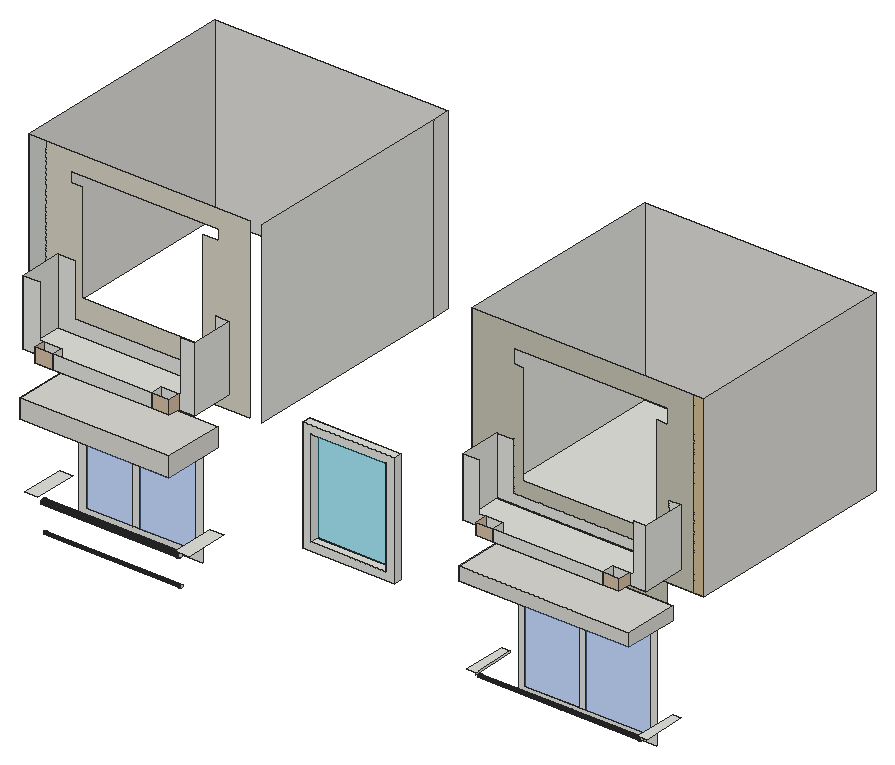
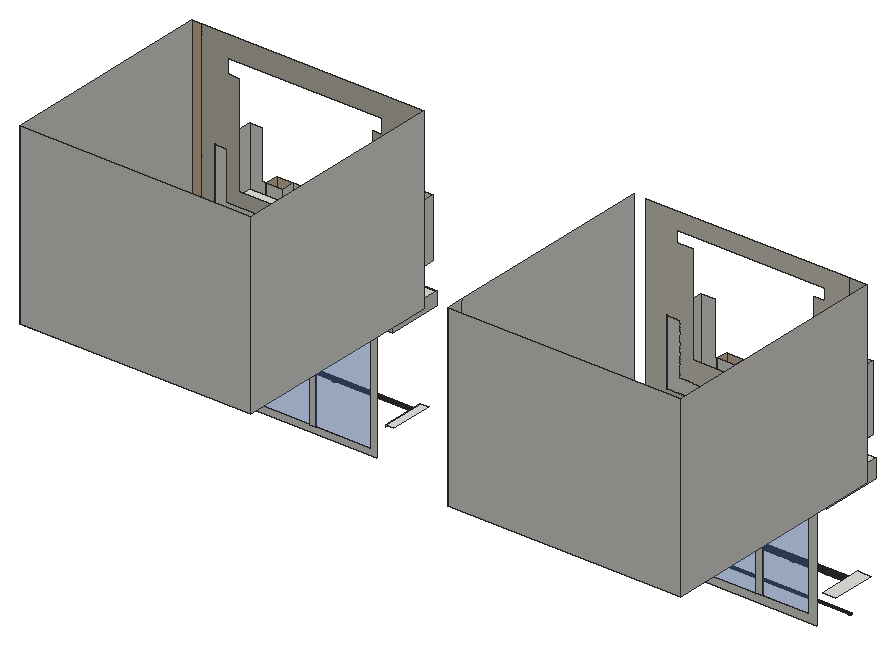
# SketchUp Ruby script. Lengths in inches.
U = 1.inch
M = Sketchup.active_model
def pt(a) = Geom::Point3d.new(a.map { |v| v * U })
def face(e, loops, mat)
  f = e.add_face(loops[0].map { |a| pt(a) })
  loops[1..].each { |l| e.add_face(l.map { |a| pt(a) }).erase! }
  f.material = f.back_material = mat if mat
  f
end
# faces: each face lists its corners as indices into pts; further lists are holes
def faces(e, pts, list, mat = nil) = list.each { |f| face(e, (f[0].is_a?(Array) ? f : [f]).map { |l| l.map { |i| pts[i] } }, mat) }
# xy, xz, yz: faces in a plane at the given z, y or x. An outline is a flat list of corners, or four numbers for a rectangle; further outlines are holes
def ring(l) = l.size == 4 ? [[l[0], l[1]], [l[2], l[1]], [l[2], l[3]], [l[0], l[3]]] : l.each_slice(2).to_a
def flat(e, list, mat, &to3) = list.each { |f| face(e, (f[0].is_a?(Array) ? f : [f]).map { |l| ring(l).map { |u, v| to3.(u, v) } }, mat) }
def xy(e, z, list, mat = nil) = flat(e, list, mat) { |x, y| [x, y, z] }
def xz(e, y, list, mat = nil) = flat(e, list, mat) { |x, z| [x, y, z] }
def yz(e, x, list, mat = nil) = flat(e, list, mat) { |y, z| [x, y, z] }
def lines(e, pts, list) = list.each { |a, b| e.add_line(pt(pts[a]), pt(pts[b])) }
# prism: a flat outline (further loops are holes) pulled along v
def prism(e, loops, v, mat = nil)
  f = face(e, loops, mat); d = Geom::Vector3d.new(v.map { |x| x * U })
  f.pushpull(f.normal.samedirection?(d) ? d.length : -d.length)
end
def box(e, o, s, mat = nil) = prism(e, [[o, [o[0] + s[0], o[1], o[2]], [o[0] + s[0], o[1] + s[1], o[2]], [o[0], o[1] + s[1], o[2]]]], [0, 0, s[2]], mat)
def at(x, y, z, deg = 0) = Geom::Transformation.translation(pt([x, y, z])) * Geom::Transformation.rotation(ORIGIN, Z_AXIS, deg.degrees)
def axes(o, x, y, z) = Geom::Transformation.new([*x, 0, *y, 0, *z, 0, *pt(o).to_a, 1])
def part(name) = M.definitions.add(name)
# library, detail: a bought-in or finely detailed component or shape, given as its bounding box
def library(name, o, s) = part(name).tap { |d| box(d.entities, o, s) }
def detail(e, o, s) = box(e.add_group.entities, o, s)
def put(e, d, t, mat = nil) = e.add_instance(d, t).tap { |i| i.material = mat if mat }
def group(e, t, mat = nil) = e.add_group.tap { |g| g.transformation = t; g.material = mat if mat }.entities
root = M.entities
M.materials.add("[Basic Tile]").color = [203, 206, 202]
M.materials.add("[Color M07]").color = [58, 58, 58]
M.materials.add("[Formica Beige]").color = [211, 187, 149]
M.materials.add("[Formica Graystone]").color = [198, 194, 180]
M.materials.add("[Formica Graystone]1").color = [216, 212, 196]
M.materials.add("[Formica Laminate Dark]").color = [50, 53, 60]
M.materials.add("[Formica Laminate Light]").color = [213, 189, 164]
M.materials.add("[Quartz Light Brown]").color = [199, 184, 152]
M.materials.add("[Terrazzo Tile Accent]").color = [224, 221, 217]
M.materials.add("[Terrazzo Tile Light]").color = [219, 217, 210]
M.materials.add("[Translucent Glass Blue]").color = [85, 126, 201]
M.materials["[Translucent Glass Blue]"].alpha = 0.5
M.materials.add("[Translucent Glass Tinted]").color = [5, 144, 173]
M.materials["[Translucent Glass Tinted]"].alpha = 0.48
xy(root,189.05,[[338.06,91.37,338.38,91.41,338.68,91.54,338.94,91.74,339.14,91.99,339.26,92.3,339.31,92.62,339.26,92.94,339.14,93.24,338.94,93.5,338.68,93.7,338.38,93.83,338.06,93.87,337.73,93.83,337.43,93.7,337.17,93.5,336.97,93.24,336.85,92.94,336.81,92.62,336.85,92.3,336.97,91.99,337.17,91.74,337.43,91.54,337.73,91.41]],"[Formica Laminate Dark]")
xy(root,189.11,[[363.84,91.61,364.02,91.64,364.1875,91.7,364.33,91.8125,364.44,91.96,364.51,92.12,364.53,92.3,364.51,92.48,364.44,92.64,364.33,92.79,364.1875,92.89,364.02,92.96,363.84,92.99,363.67,92.96,363.5,92.89,363.36,92.79,363.25,92.64,363.18,92.48,363.16,92.3,363.18,92.12,363.25,91.96,363.36,91.8125,363.5,91.7,363.67,91.64]])
xy(root,189.24,[[295.09,91.61,295.27,91.64,295.4375,91.7,295.58,91.8125,295.69,91.96,295.76,92.12,295.78,92.3,295.76,92.48,295.69,92.64,295.58,92.79,295.4375,92.89,295.27,92.96,295.09,92.99,294.92,92.96,294.75,92.89,294.61,92.79,294.5,92.64,294.43,92.48,294.41,92.3,294.43,92.12,294.5,91.96,294.61,91.8125,294.75,91.7,294.92,91.64]])
xy(root,189.36,[[306.16,91.61,306.34,91.64,306.5,91.7,306.64,91.8125,306.75,91.96,306.82,92.12,306.84,92.3,306.82,92.48,306.75,92.64,306.64,92.79,306.5,92.89,306.34,92.96,306.16,92.99,305.98,92.96,305.8125,92.89,305.67,92.79,305.5625,92.64,305.49,92.48,305.47,92.3,305.49,92.12,305.5625,91.96,305.67,91.8125,305.8125,91.7,305.98,91.64],[331.72,91.61,331.9,91.64,332.0625,91.7,332.21,91.8125,332.32,91.96,332.38,92.12,332.41,92.3,332.38,92.48,332.32,92.64,332.21,92.79,332.0625,92.89,331.9,92.96,331.72,92.99,331.54,92.96,331.375,92.89,331.23,92.79,331.125,92.64,331.06,92.48,331.03,92.3,331.06,92.12,331.125,91.96,331.23,91.8125,331.375,91.7,331.54,91.64],[369.28,91.61,369.46,91.64,369.625,91.7,369.77,91.8125,369.88,91.96,369.95,92.12,369.97,92.3,369.95,92.48,369.88,92.64,369.77,92.79,369.625,92.89,369.46,92.96,369.28,92.99,369.1,92.96,368.9375,92.89,368.8,92.79,368.6875,92.64,368.62,92.48,368.59,92.3,368.62,92.12,368.6875,91.96,368.8,91.8125,368.9375,91.7,369.1,91.64],[374.84,91.61,375.02,91.64,375.1875,91.7,375.33,91.8125,375.44,91.96,375.51,92.12,375.53,92.3,375.51,92.48,375.44,92.64,375.33,92.79,375.1875,92.89,375.02,92.96,374.84,92.99,374.67,92.96,374.5,92.89,374.36,92.79,374.25,92.64,374.18,92.48,374.16,92.3,374.18,92.12,374.25,91.96,374.36,91.8125,374.5,91.7,374.67,91.64]])
xy(root,189.41,[[79.52,92.43,79.76,92.46,79.81,92.48,79.99,92.55,80.18,92.7,80.33,92.9,80.42,93.125,80.45,93.37,80.42,93.61,80.35,93.79,80.33,93.83,80.18,94.03,79.99,94.18,79.76,94.27,79.52,94.3,79.27,94.27,79.05,94.18,78.85,94.03,78.7,93.83,78.6875,93.79,78.61,93.61,78.58,93.37,78.61,93.125,78.7,92.9,78.85,92.7,79.05,92.55,79.23,92.48,79.27,92.46]])
xy(root,189.42,[[300.84,91.61,301.02,91.64,301.1875,91.7,301.33,91.8125,301.44,91.96,301.51,92.12,301.53,92.3,301.51,92.48,301.44,92.64,301.33,92.79,301.1875,92.89,301.02,92.96,300.84,92.99,300.67,92.96,300.5,92.89,300.36,92.79,300.25,92.64,300.18,92.48,300.16,92.3,300.18,92.12,300.25,91.96,300.36,91.8125,300.5,91.7,300.67,91.64],[353.72,91.61,353.9,91.64,354.0625,91.7,354.21,91.8125,354.32,91.96,354.38,92.12,354.41,92.3,354.38,92.48,354.32,92.64,354.21,92.79,354.0625,92.89,353.9,92.96,353.72,92.99,353.54,92.96,353.375,92.89,353.23,92.79,353.125,92.64,353.06,92.48,353.03,92.3,353.06,92.12,353.125,91.96,353.23,91.8125,353.375,91.7,353.54,91.64],[378.93,91.61,379.11,91.64,379.28,91.7,379.42,91.8125,379.53,91.96,379.6,92.12,379.62,92.3,379.6,92.48,379.53,92.64,379.42,92.79,379.28,92.89,379.11,92.96,378.93,92.99,378.76,92.96,378.59,92.89,378.45,92.79,378.34,92.64,378.27,92.48,378.25,92.3,378.27,92.12,378.34,91.96,378.45,91.8125,378.59,91.7,378.76,91.64]])
xy(root,189.53,[[60.58,92.43,60.82,92.46,61.05,92.55,61.24,92.7,61.39,92.9,61.48,93.125,61.52,93.37,61.48,93.61,61.39,93.83,61.24,94.03,61.05,94.18,60.82,94.27,60.58,94.3,60.34,94.27,60.11,94.18,59.92,94.03,59.77,93.83,59.67,93.61,59.64,93.37,59.67,93.125,59.77,92.9,59.92,92.7,60.11,92.55,60.34,92.46]])
xy(root,189.6,[[55.27,92.43,55.51,92.46,55.74,92.55,55.93,92.7,56.08,92.9,56.17,93.125,56.2,93.37,56.17,93.61,56.08,93.83,55.93,94.03,55.74,94.18,55.51,94.27,55.27,94.3,55.02,94.27,54.8,94.18,54.6,94.03,54.45,93.83,54.36,93.61,54.33,93.37,54.36,93.125,54.45,92.9,54.6,92.7,54.8,92.55,55.02,92.46]])
xy(root,189.8,[[348.06,91.61,348.24,91.64,348.4,91.7,348.55,91.8125,348.65,91.96,348.72,92.12,348.75,92.3,348.72,92.48,348.65,92.64,348.55,92.79,348.4,92.89,348.24,92.96,348.06,92.99,347.88,92.96,347.72,92.89,347.57,92.79,347.46,92.64,347.4,92.48,347.37,92.3,347.4,92.12,347.46,91.96,347.57,91.8125,347.72,91.7,347.88,91.64]])
xy(root,189.8125,[[358.97,91.61,359.15,91.64,359.3125,91.7,359.46,91.8125,359.57,91.96,359.63,92.12,359.66,92.3,359.63,92.48,359.57,92.64,359.46,92.79,359.3125,92.89,359.15,92.96,358.97,92.99,358.79,92.96,358.625,92.89,358.48,92.79,358.375,92.64,358.31,92.48,358.28,92.3,358.31,92.12,358.375,91.96,358.48,91.8125,358.625,91.7,358.79,91.64]])
xy(root,189.85,[[49.7,92.43,49.95,92.46,50.17,92.55,50.37,92.7,50.52,92.9,50.61,93.125,50.64,93.37,50.61,93.61,50.52,93.83,50.37,94.03,50.17,94.18,49.95,94.27,49.7,94.3,49.46,94.27,49.24,94.18,49.04,94.03,48.89,93.83,48.8,93.61,48.77,93.37,48.8,93.125,48.89,92.9,49.04,92.7,49.24,92.55,49.46,92.46],[67.02,92.43,67.26,92.46,67.49,92.55,67.68,92.7,67.83,92.9,67.92,93.125,67.95,93.37,67.92,93.61,67.83,93.83,67.68,94.03,67.49,94.18,67.26,94.27,67.02,94.3,66.77,94.27,66.55,94.18,66.35,94.03,66.2,93.83,66.11,93.61,66.08,93.37,66.11,93.125,66.2,92.9,66.35,92.7,66.55,92.55,66.77,92.46]])
xy(root,189.86,[[317.59,91.61,317.77,91.64,317.9375,91.7,318.08,91.8125,318.19,91.96,318.26,92.12,318.28,92.3,318.26,92.48,318.19,92.64,318.08,92.79,317.9375,92.89,317.77,92.96,317.59,92.99,317.42,92.96,317.25,92.89,317.11,92.79,317,92.64,316.93,92.48,316.91,92.3,316.93,92.12,317,91.96,317.11,91.8125,317.25,91.7,317.42,91.64]])
xy(root,189.97,[[105.33,92.43,105.57,92.46,105.8,92.55,105.99,92.7,106.14,92.9,106.23,93.125,106.27,93.37,106.23,93.61,106.14,93.83,105.99,94.03,105.8,94.18,105.57,94.27,105.33,94.3,105.09,94.27,104.86,94.18,104.67,94.03,104.52,93.83,104.42,93.61,104.39,93.37,104.42,93.125,104.52,92.9,104.67,92.7,104.86,92.55,105.09,92.46]])
xy(root,190.01,[[324.09,91.61,324.27,91.64,324.4,91.6875,323.79,91.6875,323.92,91.64],[323.79,91.6875,324.4,91.6875,324.4375,91.7,324.58,91.8125,324.69,91.96,324.76,92.12,324.78,92.3,324.76,92.48,324.69,92.64,324.58,92.79,324.4375,92.89,324.27,92.96,324.09,92.99,323.92,92.96,323.75,92.89,323.61,92.79,323.5,92.64,323.43,92.48,323.41,92.3,323.43,92.12,323.5,91.96,323.61,91.8125,323.75,91.7],[343.15,91.6875,344.15,91.6875,344.31,91.8125,344.46,92.01,344.56,92.23,344.59,92.47,344.56,92.72,344.46,92.94,344.35,93.09,342.96,93.09,342.84,92.94,342.75,92.72,342.71,92.47,342.75,92.23,342.84,92.01,342.99,91.8125]])
xy(root,190.01,[[343.65,91.54,343.89,91.57,344.12,91.66,344.15,91.6875,343.15,91.6875,343.18,91.66,343.41,91.57],[342.96,93.09,344.35,93.09,344.31,93.14,344.12,93.29,343.89,93.38,343.65,93.41,343.41,93.38,343.18,93.29,342.99,93.14]],"[Formica Laminate Dark]")
xy(root,190.03,[[86.23,92.1,86.57,92.15,86.89,92.28,87.16,92.48,87.37,92.76,87.5,93.07,87.54,93.41,87.5,93.75,87.37,94.07,87.16,94.34,86.89,94.55,86.57,94.68,86.23,94.73,85.89,94.68,85.57,94.55,85.3,94.34,85.09,94.07,84.96,93.75,84.92,93.41,84.96,93.07,85.09,92.76,85.3,92.48,85.57,92.28,85.89,92.15]])
xy(root,190.1,[[112.45,92.43,112.7,92.46,112.92,92.55,113.12,92.7,113.27,92.9,113.36,93.125,113.39,93.37,113.36,93.61,113.27,93.83,113.12,94.03,112.92,94.18,112.7,94.27,112.45,94.3,112.21,94.27,111.99,94.18,111.79,94.03,111.64,93.83,111.55,93.61,111.52,93.37,111.55,93.125,111.64,92.9,111.79,92.7,111.99,92.55,112.21,92.46]])
xy(root,190.11,[[312.78,91.61,312.96,91.64,313.125,91.7,313.27,91.8125,313.38,91.96,313.45,92.12,313.47,92.3,313.45,92.48,313.38,92.64,313.27,92.79,313.125,92.89,312.96,92.96,312.78,92.99,312.6,92.96,312.4375,92.89,312.3,92.79,312.1875,92.64,312.12,92.48,312.09,92.3,312.12,92.12,312.1875,91.96,312.3,91.8125,312.4375,91.7,312.6,91.64]])
xy(root,190.22,[[118.7,92.43,118.95,92.46,119.17,92.55,119.37,92.7,119.52,92.9,119.61,93.125,119.64,93.37,119.61,93.61,119.52,93.83,119.37,94.03,119.17,94.18,118.95,94.27,118.7,94.3,118.46,94.27,118.24,94.18,118.04,94.03,117.89,93.83,117.8,93.61,117.77,93.37,117.8,93.125,117.89,92.9,118.04,92.7,118.24,92.55,118.46,92.46]])
xy(root,190.41,[[98.64,92.43,98.88,92.46,99.11,92.55,99.3,92.7,99.45,92.9,99.55,93.125,99.58,93.37,99.55,93.61,99.45,93.83,99.3,94.03,99.11,94.18,98.88,94.27,98.64,94.3,98.4,94.27,98.17,94.18,97.98,94.03,97.83,93.83,97.74,93.61,97.7,93.37,97.74,93.125,97.83,92.9,97.98,92.7,98.17,92.55,98.4,92.46]])
xy(root,190.53,[[92.58,92.43,92.82,92.46,93.05,92.55,93.24,92.7,93.39,92.9,93.48,93.125,93.52,93.37,93.48,93.61,93.39,93.83,93.24,94.03,93.05,94.18,92.82,94.27,92.58,94.3,92.34,94.27,92.11,94.18,91.92,94.03,91.77,93.83,91.67,93.61,91.64,93.37,91.67,93.125,91.77,92.9,91.92,92.7,92.11,92.55,92.34,92.46]])
xy(root,190.89,[[73.27,92.43,73.51,92.46,73.74,92.55,73.93,92.7,74.08,92.9,74.17,93.125,74.2,93.37,74.17,93.61,74.08,93.83,73.93,94.03,73.74,94.18,73.51,94.27,73.27,94.3,73.02,94.27,72.8,94.18,72.6,94.03,72.45,93.83,72.36,93.61,72.33,93.37,72.36,93.125,72.45,92.9,72.6,92.7,72.8,92.55,73.02,92.46]])
xy(root,192.125,[[287.34,89.73,292.1875,114.1],[383.79,89.73,388.41,114.1]])
xy(root,194.03,[[38.84,89.73,46.18,114.1],[123.57,89.73,131.22,114.1]])
xy(root,206.5625,[[179.41,109.54,230.79,114.1]])
xy(root,211.17,[[184.02,109.54,226.18,114.1]])
xy(root,234.18,[[49.84,107.79,119.34,114.1]],"[Quartz Light Brown]")
xy(root,235.5625,[[49.84,107.79,119.34,109.6],[49.84,109.6,119.34,114.1]])
xy(root,236.95,[[49.84,109.6,119.34,114.1]])
xy(root,236.95,[[[43.93,79.73,43.93,114.1,49.84,114.1,49.84,109.6,119.34,109.6,119.34,114.1,128,114.1,128,79.73],[54.42,83.75,54.97,83.82,55.49,84.04,55.93,84.375,56.26,84.81,56.48,85.33,56.55,85.88,56.48,86.43,56.26,86.94,55.93,87.38,55.49,87.72,54.97,87.93,54.42,88,53.87,87.93,53.36,87.72,52.92,87.38,52.58,86.94,52.37,86.43,52.3,85.88,52.37,85.33,52.58,84.81,52.92,84.375,53.36,84.04,53.87,83.82],[116.8,83.75,117.35,83.82,117.86,84.04,118.3,84.375,118.64,84.81,118.85,85.33,118.92,85.88,118.85,86.43,118.64,86.94,118.3,87.38,117.86,87.72,117.35,87.93,116.8,88,116.25,87.93,115.74,87.72,115.3,87.38,114.96,86.94,114.75,86.43,114.67,85.88,114.75,85.33,114.96,84.81,115.3,84.375,115.74,84.04,116.25,83.82]]],"[Terrazzo Tile Light]")
xy(root,239.81,[[[288.22,83.29,383.91,114.1],[298.91,84.16,299.52,84.16,300.1,84.31,300.63,84.6,301.06,85.02,301.37,85.54,301.53,86.125,301.54,86.73,301.39,87.3125,301.09,87.84,300.67,88.27,300.15,88.58,299.57,88.74,298.97,88.75,298.38,88.6,297.86,88.3,297.42,87.88,297.12,87.36,296.95,86.78,296.95,86.18,297.09,85.59,297.39,85.07,297.8125,84.63,298.33,84.33],[376.35,84.16,376.95,84.16,377.54,84.31,378.07,84.6,378.5,85.02,378.81,85.54,378.97,86.125,378.98,86.73,378.83,87.3125,378.53,87.84,378.11,88.27,377.59,88.58,377.01,88.74,376.4,88.75,375.82,88.6,375.29,88.3,374.86,87.88,374.55,87.36,374.39,86.78,374.38,86.18,374.53,85.59,374.83,85.07,375.25,84.63,375.77,84.33]]],"[Terrazzo Tile Light]")
xy(root,247.3125,[[288.22,83.29,383.91,114.1]],"[Terrazzo Tile Light]")
xy(root,247.76,[[43.93,79.73,128,114.1]],"[Terrazzo Tile Light]")
xy(root,258,[[270.97,114.1,401.16,235.11]])
xy(root,265.65,[[184.02,109.54,226.18,114.1]])
xy(root,265.89,[[59.49,83.35,59.49,89.73,37.87,89.73,37.87,114.1,134.24,114.1,134.24,89.73,115.23,89.73,115.23,83.35]])
xy(root,265.89,[[49.6,83.35,59.49,89.73],[115.23,83.35,125.11,89.73]],"[Formica Laminate Light]")
xy(root,266.68,[[307.63,82.54,307.63,89.73,284.91,89.73,284.91,114.1,388.23,114.1,388.23,89.73,369.37,89.73,369.37,82.54]])
xy(root,266.68,[[298.18,82.54,307.63,89.73],[369.37,82.54,378.82,89.73]],"[Formica Laminate Light]")
xy(root,270.25,[[179.41,109.54,230.79,114.1]])
xz(root,79.73,[[43.93,236.95,128,247.76]],"[Terrazzo Tile Light]")
xz(root,82.54,[[307.63,266.68,369.37,272.93]])
xz(root,82.54,[[298.18,266.68,307.63,272.93],[369.37,266.68,378.82,272.93]],"[Formica Laminate Light]")
xz(root,83.29,[[288.22,239.81,383.91,247.3125]],"[Terrazzo Tile Light]")
xz(root,83.35,[[59.49,265.89,115.23,273.71]])
xz(root,83.35,[[49.6,265.89,59.49,273.71],[115.23,265.89,125.11,273.71]],"[Formica Laminate Light]")
xz(root,89.73,[[37.87,265.89,49.6,265.89,49.6,273.71,47.16,273.71,47.16,302.83,37.87,302.83],[49.6,265.89,59.49,273.71],[115.23,265.89,125.11,273.71],[125.11,265.89,134.24,265.89,134.24,302.83,126.66,302.83,126.66,273.71,125.11,273.71],[284.91,266.68,298.18,266.68,298.18,272.93,294.34,272.93,294.34,299.8,284.91,299.8],
  [298.18,266.68,307.63,272.93],[369.37,266.68,378.82,272.93],[378.82,266.68,388.23,266.68,388.23,299.8,381.41,299.8,381.41,272.93,378.82,272.93]])
xz(root,107.79,[[49.84,234.18,119.34,235.5625]],"[Quartz Light Brown]")
xz(root,109.54,[[[179.41,206.5625,230.79,270.25],[184.02,211.17,226.18,265.65]]])
xz(root,109.6,[[49.84,235.5625,119.34,236.95]],"[Quartz Light Brown]")
xz(root,114.1,[[[297.03,173.62,374.84,239.81],[300.64,177.23,371.24,236.2]],[[49.84,176.18,119.34,234.18],[53.96,180.3,115.22,232.62]],[331.67,177.23,335,236.2],[80.25,180.3,83.94,232.62],[[179.41,206.5625,230.79,270.25],[184.02,211.17,226.18,265.65]],
  [49.84,234.18,119.34,235.5625],[49.84,235.5625,119.34,236.95],[288.22,239.81,383.91,247.3125],[37.87,265.89,37.87,302.83,47.16,302.83,47.16,273.71,126.66,273.71,126.66,302.83,134.24,302.83,134.24,265.89],[284.91,266.68,284.91,299.8,294.34,299.8,294.34,272.93,381.41,272.93,381.41,299.8,388.23,299.8,388.23,266.68]])
xz(root,114.1,[[21.57,258,31.29,357.6875]],"[Basic Tile]")
xz(root,114.1,[[395.49,258,401.16,357.6875]],"[Formica Beige]")
xz(root,114.1,[[288.22,247.3125,380.22,258],[[270.97,258,395.49,357.6875],[299.6,280.54,299.6,337.71,294.42,337.71,294.42,345.83,381.23,345.83,381.23,337.71,374.79,337.71,374.79,280.54],[284.91,266.68,284.91,299.8,294.34,299.8,294.34,272.93,381.41,272.93,381.41,299.8,388.23,299.8,388.23,266.68]]],"[Formica Graystone]")
xz(root,114.1,[[[31.29,258,145.58,357.6875],[51.12,285.36,51.12,341.31,45.36,341.31,45.36,347.68,128.55,347.68,128.55,341.31,119.37,341.31,119.37,285.36],[37.87,265.89,37.87,302.83,47.16,302.83,47.16,273.71,126.66,273.71,126.66,302.83,134.24,302.83,134.24,265.89]]],"[Formica Graystone]1")
xz(root,114.1,[[300.64,177.23,331.67,236.2],[335,177.23,371.24,236.2],[53.96,180.3,80.25,232.62],[83.94,180.3,115.22,232.62]],"[Translucent Glass Blue]")
xz(root,114.1,[[184.02,211.17,226.18,265.65]],"[Translucent Glass Tinted]")
xz(root,235.11,[[270.97,258,401.16,357.6875]],"[Terrazzo Tile Accent]")
xz(root,244.83,[[21.57,258,152.39,357.6875]],"[Terrazzo Tile Accent]")
yz(root,21.57,[[114.1,258,244.83,357.6875]],"[Terrazzo Tile Accent]")
yz(root,37.87,[[89.73,265.89,114.1,302.83]])
yz(root,43.93,[[79.73,236.95,114.1,247.76]],"[Terrazzo Tile Light]")
yz(root,49.6,[[83.35,265.89,89.73,273.71]],"[Formica Laminate Light]")
yz(root,49.84,[[107.79,234.18,114.1,235.5625],[109.6,235.5625,114.1,236.95]],"[Quartz Light Brown]")
yz(root,59.49,[[83.35,265.89,89.73,273.71]])
yz(root,115.23,[[83.35,265.89,89.73,273.71]])
yz(root,119.34,[[107.79,234.18,114.1,235.5625],[109.6,235.5625,114.1,236.95]],"[Quartz Light Brown]")
yz(root,123.57,[[94.01,173.9,94.15,173.92,94.29,173.98,94.41,174.07,94.5,174.18,94.55,174.32,94.57,174.47,94.55,174.61,94.5,174.75,94.41,174.86,94.29,174.95,94.15,175.01,94.01,175.03,93.86,175.01,93.73,174.95,93.61,174.86,93.52,174.75,93.47,174.61,93.45,174.47,93.47,174.32,93.52,174.18,93.61,174.07,93.73,173.98,93.86,173.92],[93.14,189.23,93.48,189.28,93.79,189.41,94.06,189.62,94.27,189.89,94.4,190.21,94.45,190.55,94.4,190.89,94.27,191.2,94.06,191.47,93.79,191.68,93.48,191.81,93.14,191.86,92.8,191.81,92.48,191.68,92.21,191.47,92,191.2,91.87,190.89,91.82,190.55,91.87,190.21,92,189.89,92.21,189.62,92.48,189.41,92.8,189.28]])
yz(root,125.11,[[83.35,265.89,89.73,273.71]],"[Formica Laminate Light]")
yz(root,128,[[79.73,236.95,114.1,247.76]],"[Terrazzo Tile Light]")
yz(root,134.24,[[89.73,265.89,114.1,302.83]])
yz(root,152.39,[[114.1,258,235.11,357.6875]])
yz(root,152.39,[[235.11,258,244.83,357.6875]],"[Terrazzo Tile Accent]")
yz(root,179.41,[[109.54,206.5625,114.1,270.25]])
yz(root,184.02,[[109.54,211.17,114.1,265.65]])
yz(root,226.18,[[109.54,211.17,114.1,265.65]])
yz(root,230.79,[[109.54,206.5625,114.1,270.25]])
yz(root,270.97,[[114.1,258,235.11,357.6875]])
yz(root,284.91,[[89.73,266.68,114.1,299.8]])
yz(root,288.22,[[83.29,239.81,114.1,247.3125]],"[Terrazzo Tile Light]")
yz(root,292.1875,[[89.73,191.16,114.1,192.125]])
yz(root,298.18,[[82.54,266.68,89.73,272.93]],"[Formica Laminate Light]")
yz(root,307.63,[[82.54,266.68,89.73,272.93]])
yz(root,369.37,[[82.54,266.68,89.73,272.93]])
yz(root,378.82,[[82.54,266.68,89.73,272.93]],"[Formica Laminate Light]")
yz(root,383.79,[[92.39,188.79,92.6,188.82,92.8,188.9,92.96,189.03,93.09,189.2,93.18,189.39,93.2,189.6,93.18,189.8125,93.09,190.01,92.96,190.18,92.8,190.31,92.6,190.39,92.39,190.42,92.18,190.39,91.98,190.31,91.82,190.18,91.6875,190.01,91.61,189.8125,91.58,189.6,91.61,189.39,91.6875,189.2,91.82,189.03,91.98,188.9,92.18,188.82]])
yz(root,383.91,[[83.29,239.81,114.1,247.3125]],"[Terrazzo Tile Light]")
yz(root,388.23,[[89.73,266.68,114.1,299.8]])
yz(root,401.16,[[114.1,258,235.11,357.6875]],"[Terrazzo Tile Accent]")
p = [[123.57,93.86,173.92],[123.57,93.73,173.98],[46.18,93.73,173.98],[46.18,93.86,173.92],[123.57,94.01,173.9],[46.18,94.01,173.9],
  [123.57,94.15,173.92],[46.18,94.15,173.92],[123.57,94.29,173.98],[46.18,94.29,173.98],[123.57,93.61,174.07],[46.18,93.61,174.07],
  [123.57,94.41,174.07],[46.18,94.41,174.07],[123.57,93.52,174.18],[46.18,93.52,174.18],[123.57,94.5,174.18],[46.18,94.5,174.18],
  [123.57,93.47,174.32],[46.18,93.47,174.32],[123.57,94.55,174.32],[46.18,94.55,174.32],[123.57,93.45,174.47],[46.18,93.45,174.47],
  [123.57,94.57,174.47],[46.18,94.57,174.47],[123.57,93.47,174.61],[46.18,93.47,174.61],[123.57,94.55,174.61],[46.18,94.55,174.61],
  [123.57,93.52,174.75],[46.18,93.52,174.75],[123.57,94.5,174.75],[46.18,94.5,174.75],[123.57,93.61,174.86],[46.18,93.61,174.86],
  [123.57,94.41,174.86],[46.18,94.41,174.86],[123.57,93.73,174.95],[46.18,93.73,174.95],[123.57,94.29,174.95],[46.18,94.29,174.95],
  [123.57,93.86,175.01],[46.18,93.86,175.01],[123.57,94.01,175.03],[46.18,94.01,175.03],[123.57,94.15,175.01],[46.18,94.15,175.01],
  [383.79,92.18,188.82],[383.79,91.98,188.9],[292.1875,91.98,188.9],[292.1875,92.18,188.82],[383.79,92.39,188.79],[292.1875,92.39,188.79],
  [383.79,92.6,188.82],[292.1875,92.6,188.82],[383.79,92.8,188.9],[292.1875,92.8,188.9],[383.79,91.82,189.03],[292.1875,91.82,189.03],
  [383.79,92.96,189.03],[292.1875,92.96,189.03],[383.79,91.6875,189.2],[292.1875,91.6875,189.2],[383.79,93.09,189.2],[292.1875,93.09,189.2],
  [383.79,91.61,189.39],[292.1875,91.61,189.39],[123.57,93.14,189.23],[123.57,92.8,189.28],[46.18,92.8,189.28],[46.18,93.14,189.23],
  [123.57,93.48,189.28],[46.18,93.48,189.28],[383.79,93.18,189.39],[292.1875,93.18,189.39],[123.57,92.48,189.41],[79.81,92.48,189.41],
  [79.23,92.48,189.41],[46.18,92.48,189.41],[123.57,93.79,189.41],[46.18,93.79,189.41],[78.6875,93.79,189.41],[80.35,93.79,189.41],
  [383.79,91.58,189.6],[292.1875,91.58,189.6],[123.57,92.21,189.62],[46.18,92.21,189.62],[383.79,93.2,189.6],[292.1875,93.2,189.6],
  [123.57,94.06,189.62],[46.18,94.06,189.62],[383.79,91.61,189.8125],[292.1875,91.61,189.8125],[123.57,92,189.89],[46.18,92,189.89],
  [383.79,93.18,189.8125],[292.1875,93.18,189.8125],[123.57,94.27,189.89],[46.18,94.27,189.89],[383.79,91.6875,190.01],[344.15,91.6875,190.01],
  [343.15,91.6875,190.01],[324.4,91.6875,190.01],[323.79,91.6875,190.01],[292.1875,91.6875,190.01],[383.79,93.09,190.01],[292.1875,93.09,190.01],
  [342.96,93.09,190.01],[344.35,93.09,190.01],[123.57,91.87,190.21],[46.18,91.87,190.21],[123.57,94.4,190.21],[46.18,94.4,190.21],
  [383.79,91.82,190.18],[292.1875,91.82,190.18],[383.79,92.96,190.18],[292.1875,92.96,190.18],[123.57,91.82,190.55],[46.18,91.82,190.55],
  [383.79,91.98,190.31],[292.1875,91.98,190.31],[383.79,92.8,190.31],[292.1875,92.8,190.31],[123.57,94.45,190.55],[46.18,94.45,190.55],
  [383.79,92.18,190.39],[292.1875,92.18,190.39],[383.79,92.6,190.39],[292.1875,92.6,190.39],[383.79,92.39,190.42],[292.1875,92.39,190.42],
  [123.57,91.87,190.89],[46.18,91.87,190.89],[123.57,94.4,190.89],[46.18,94.4,190.89],[123.57,92,191.2],[46.18,92,191.2],
  [123.57,94.27,191.2],[46.18,94.27,191.2],[123.57,92.21,191.47],[46.18,92.21,191.47],[123.57,94.06,191.47],[46.18,94.06,191.47],
  [123.57,92.48,191.68],[46.18,92.48,191.68],[123.57,93.79,191.68],[46.18,93.79,191.68],[123.57,92.8,191.81],[46.18,92.8,191.81],
  [123.57,93.48,191.81],[46.18,93.48,191.81],[123.57,93.14,191.86],[46.18,93.14,191.86]]
faces(root,p,[[0,1,2,3],[4,0,3,5],[6,4,5,7],[8,6,7,9],[1,10,11,2],[12,8,9,13],[10,14,15,11],[16,12,13,17],
  [14,18,19,15],[20,16,17,21],[18,22,23,19],[24,20,21,25],[22,26,27,23],[28,24,25,29],[26,30,31,27],[32,28,29,33],
  [30,34,35,31],[36,32,33,37],[34,38,39,35],[40,36,37,41],[38,42,43,39],[42,44,45,43],[44,46,47,45],[46,40,41,47],
  [68,69,70,71],[72,68,71,73],[69,76,77,78,79,70],[80,72,73,81,82,83],[76,86,87,79,78,77],[90,80,83,82,81,91],[86,94,95,87],[98,90,91,99],
  [94,110,111,95],[112,98,99,113],[110,118,119,111],[124,112,113,125],[118,132,133,119],[134,124,125,135],[132,136,137,133],[138,134,135,139],
  [136,140,141,137],[142,138,139,143],[140,144,145,141],[146,142,143,147],[144,148,149,145],[150,146,147,151],[148,152,153,149],[152,150,151,153]],"[Color M07]")
faces(root,p,[[48,49,50,51],[52,48,51,53],[54,52,53,55],[56,54,55,57],[49,58,59,50],[60,56,57,61],[58,62,63,59],[64,60,61,65],
  [62,66,67,63],[74,64,65,75],[66,84,85,67],[88,74,75,89],[84,92,93,85],[96,88,89,97],[92,100,101,102,103,104,105,93],[106,96,97,107,108,109],
  [100,114,115,105,104,103,102,101],[116,106,109,108,107,117],[114,120,121,115],[122,116,117,123],[120,126,127,121],[128,122,123,129],[126,130,131,127],[130,128,129,131]],"[Formica Laminate Dark]")
